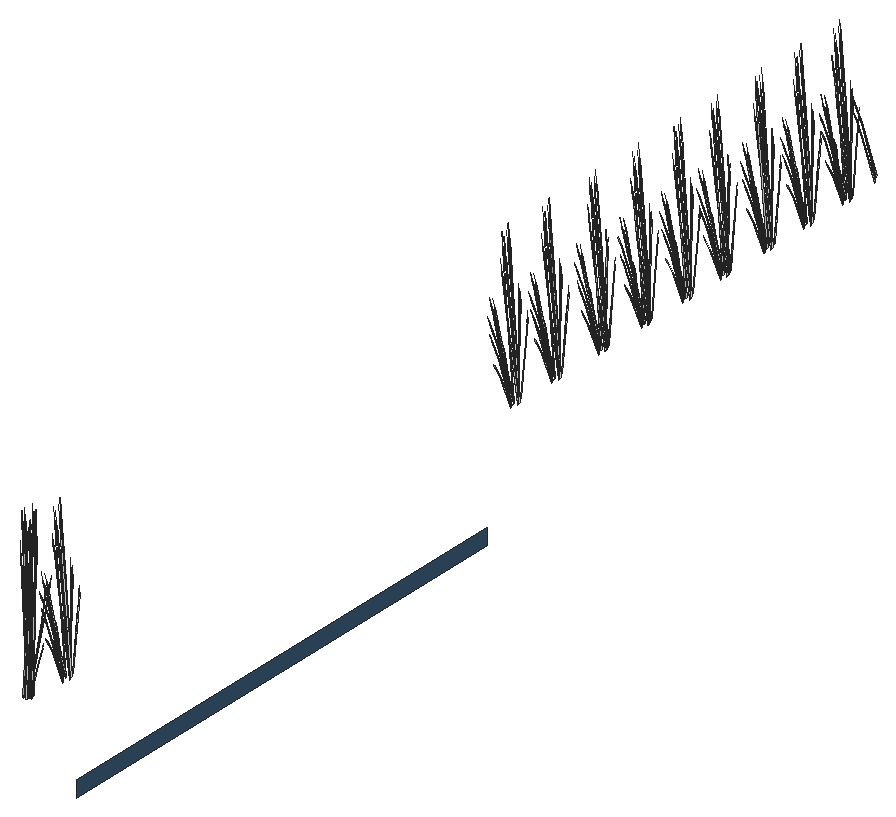
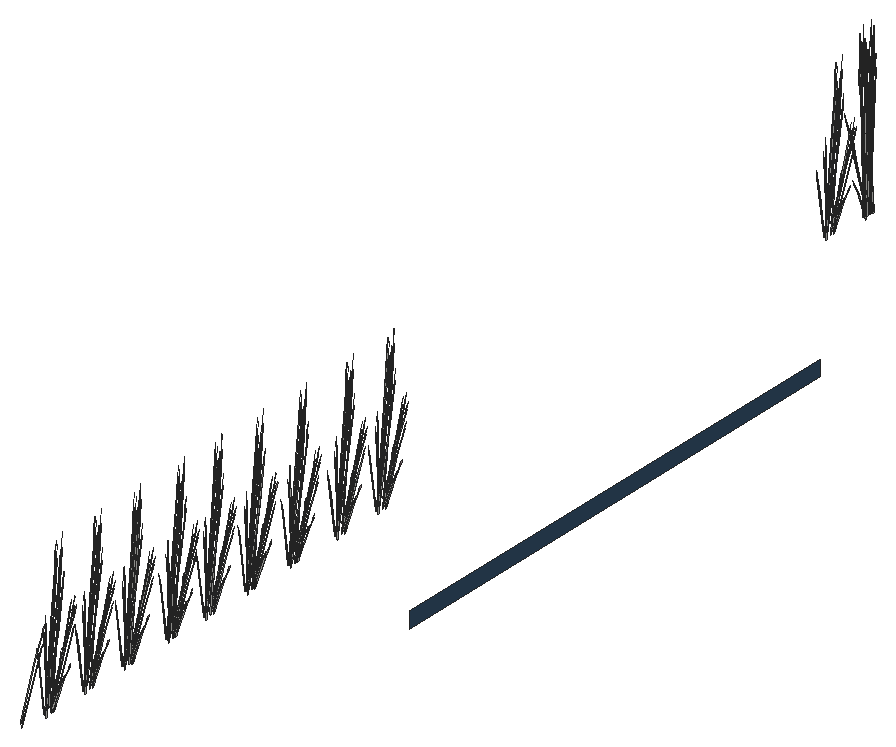
# SketchUp Ruby script. Lengths in inches.
U = 1.inch
M = Sketchup.active_model
def pt(a) = Geom::Point3d.new(a.map { |v| v * U })
def face(e, loops, mat)
  f = e.add_face(loops[0].map { |a| pt(a) })
  loops[1..].each { |l| e.add_face(l.map { |a| pt(a) }).erase! }
  f.material = f.back_material = mat if mat
  f
end
# faces: each face lists its corners as indices into pts; further lists are holes
def faces(e, pts, list, mat = nil) = list.each { |f| face(e, (f[0].is_a?(Array) ? f : [f]).map { |l| l.map { |i| pts[i] } }, mat) }
# xy, xz, yz: faces in a plane at the given z, y or x. An outline is a flat list of corners, or four numbers for a rectangle; further outlines are holes
def ring(l) = l.size == 4 ? [[l[0], l[1]], [l[2], l[1]], [l[2], l[3]], [l[0], l[3]]] : l.each_slice(2).to_a
def flat(e, list, mat, &to3) = list.each { |f| face(e, (f[0].is_a?(Array) ? f : [f]).map { |l| ring(l).map { |u, v| to3.(u, v) } }, mat) }
def xy(e, z, list, mat = nil) = flat(e, list, mat) { |x, y| [x, y, z] }
def xz(e, y, list, mat = nil) = flat(e, list, mat) { |x, z| [x, y, z] }
def yz(e, x, list, mat = nil) = flat(e, list, mat) { |y, z| [x, y, z] }
def lines(e, pts, list) = list.each { |a, b| e.add_line(pt(pts[a]), pt(pts[b])) }
# prism: a flat outline (further loops are holes) pulled along v
def prism(e, loops, v, mat = nil)
  f = face(e, loops, mat); d = Geom::Vector3d.new(v.map { |x| x * U })
  f.pushpull(f.normal.samedirection?(d) ? d.length : -d.length)
end
def box(e, o, s, mat = nil) = prism(e, [[o, [o[0] + s[0], o[1], o[2]], [o[0] + s[0], o[1] + s[1], o[2]], [o[0], o[1] + s[1], o[2]]]], [0, 0, s[2]], mat)
def at(x, y, z, deg = 0) = Geom::Transformation.translation(pt([x, y, z])) * Geom::Transformation.rotation(ORIGIN, Z_AXIS, deg.degrees)
def axes(o, x, y, z) = Geom::Transformation.new([*x, 0, *y, 0, *z, 0, *pt(o).to_a, 1])
def part(name) = M.definitions.add(name)
# library, detail: a bought-in or finely detailed component or shape, given as its bounding box
def library(name, o, s) = part(name).tap { |d| box(d.entities, o, s) }
def detail(e, o, s) = box(e.add_group.entities, o, s)
def put(e, d, t, mat = nil) = e.add_instance(d, t).tap { |i| i.material = mat if mat }
def group(e, t, mat = nil) = e.add_group.tap { |g| g.transformation = t; g.material = mat if mat }.entities
root = M.entities
M.materials.add("Carpet_04_1K").color = [56, 85, 112]
M.materials.add("LightPink_Translucent").color = [144, 107, 117]
M.materials["LightPink_Translucent"].alpha = 0.75
c1 = part("blade")
p = [[2.15,0.21,22],[0,0.17,0],[0.09,0.45,0],[2.18,0.31,22],[2.29,0.31,22],[0.38,0.45,0],
  [2.48,0.24,33],[2.49,0.24,33],[2.48,0.22,33]]
faces(c1.entities,p,[[0,1,2,3],[4,5,2,3],[6,3,4,7],[8,0,3,6]])
c2 = part("seeds")
p = [[0.3,-0.1,1.38],[-0.01,-0.03,1.59],[-0.01,-0.03,0.03],[0.14,-0.07,-0.07],[0.29,-0.03,3],[0.15,0.01,3.11]]
faces(c2.entities,p,[[0,1,2,3],[1,0,4,5]],"LightPink_Translucent")
c3 = part("blade with seeds")
put(c3.entities,c1,at(0,0,0))
put(c3.entities,c2,axes([2.4,0.25,30.99],[1.5799,-0.05474,1.17369],[-0.12525,1.92788,0.29478],[-0.07173,-0.02425,1.56792]))
yz(root,398.57,[[316.3,-42,509.26,-36]],"Carpet_04_1K")
put(root,c3,axes([400.43,618.83,4.53],[-0.30722,0.06665,-0.35414],[-0.08112,-0.381,0.4572],[-0.08804,0.10234,0.87481]))
put(root,c3,axes([400.43,639.36,4.53],[-0.30722,0.06665,-0.35414],[-0.08112,-0.381,0.4572],[-0.08804,0.10234,0.87481]))
put(root,c3,axes([400.43,658.04,4.53],[-0.30722,0.06665,-0.35414],[-0.08112,-0.381,0.4572],[-0.08804,0.10234,0.87481]))
put(root,c3,axes([400.43,676.25,4.53],[-0.30722,0.06665,-0.35414],[-0.08112,-0.381,0.4572],[-0.08804,0.10234,0.87481]))
put(root,c3,axes([398.73,292.91,2.72],[-0.17124,0.42022,0.44739],[-0.35581,-0.20224,-0.21531],[0,-0.09687,1.43643]))
put(root,c3,axes([400.27,311.16,1.49],[0.04734,0.04659,1.76342],[0.08027,0.4317,-0.26939],[-0.10492,0.09206,0.30037]))
put(root,c3,axes([400.27,521.6,1.49],[0.04734,0.04659,1.76342],[0.08027,0.4317,-0.26939],[-0.10492,0.09206,0.30037]))
put(root,c3,axes([400.27,540.83,1.49],[0.04734,0.04659,1.76342],[0.08027,0.4317,-0.26939],[-0.10492,0.09206,0.30037]))
put(root,c3,axes([400.27,562.67,1.49],[0.04734,0.04659,1.76342],[0.08027,0.4317,-0.26939],[-0.10492,0.09206,0.30037]))
put(root,c3,axes([400.27,582.9375,1.49],[0.04734,0.04659,1.76342],[0.08027,0.4317,-0.26939],[-0.10492,0.09206,0.30037]))
put(root,c3,axes([400.27,602.375,1.49],[0.04734,0.04659,1.76342],[0.08027,0.4317,-0.26939],[-0.10492,0.09206,0.30037]))
put(root,c3,axes([400.27,619.96,1.49],[0.04734,0.04659,1.76342],[0.08027,0.4317,-0.26939],[-0.10492,0.09206,0.30037]))
put(root,c3,axes([400.27,640.49,1.49],[0.04734,0.04659,1.76342],[0.08027,0.4317,-0.26939],[-0.10492,0.09206,0.30037]))
put(root,c3,axes([400.27,659.17,1.49],[0.04734,0.04659,1.76342],[0.08027,0.4317,-0.26939],[-0.10492,0.09206,0.30037]))
put(root,c3,axes([400.27,677.38,1.49],[0.04734,0.04659,1.76342],[0.08027,0.4317,-0.26939],[-0.10492,0.09206,0.30037]))
put(root,c3,axes([400.2,308.625,2.77],[0.22533,-0.03337,1.1486],[-0.14293,0.29403,0.84392],[-0.11135,-0.04411,0.25299]))
put(root,c3,axes([400.2,519.06,2.77],[0.22533,-0.03337,1.1486],[-0.14293,0.29403,0.84392],[-0.11135,-0.04411,0.25299]))
put(root,c3,axes([400.2,538.29,2.77],[0.22533,-0.03337,1.1486],[-0.14293,0.29403,0.84392],[-0.11135,-0.04411,0.25299]))
put(root,c3,axes([400.2,560.13,2.77],[0.22533,-0.03337,1.1486],[-0.14293,0.29403,0.84392],[-0.11135,-0.04411,0.25299]))
put(root,c3,axes([400.2,580.4,2.77],[0.22533,-0.03337,1.1486],[-0.14293,0.29403,0.84392],[-0.11135,-0.04411,0.25299]))
put(root,c3,axes([400.2,599.84,2.77],[0.22533,-0.03337,1.1486],[-0.14293,0.29403,0.84392],[-0.11135,-0.04411,0.25299]))
put(root,c3,axes([400.2,617.42,2.77],[0.22533,-0.03337,1.1486],[-0.14293,0.29403,0.84392],[-0.11135,-0.04411,0.25299]))
put(root,c3,axes([400.2,637.95,2.77],[0.22533,-0.03337,1.1486],[-0.14293,0.29403,0.84392],[-0.11135,-0.04411,0.25299]))
put(root,c3,axes([400.2,656.63,2.77],[0.22533,-0.03337,1.1486],[-0.14293,0.29403,0.84392],[-0.11135,-0.04411,0.25299]))
put(root,c3,axes([400.2,674.84,2.77],[0.22533,-0.03337,1.1486],[-0.14293,0.29403,0.84392],[-0.11135,-0.04411,0.25299]))
put(root,c3,axes([398.61,293.9,2.47],[0.37926,-0.12378,0.17642],[0.09365,0.46065,0.35086],[-0.03382,-0.06712,1.60407]))
put(root,c3,axes([399.1,293.98,2.2],[-0.35581,-0.20937,0],[0.17124,-0.43505,0],[0,0,1.62707]))
put(root,c3,axes([399.92,294.5,2.375],[0.22066,0.46731,0],[-0.36918,0.26061,-0.51607],[-0.08408,0.05936,1.63711]))
put(root,c3,axes([399.74,293.93,2.47],[0.10196,-0.46348,0.17642],[0.3731,0.13116,0.35086],[-0.06445,0.00226,1.60407]))
put(root,c3,axes([400.9,310.01,3.875],[0.06572,-0.16029,1.71376],[0.27569,0.33172,0.13857],[-0.12437,0.20675,0.73262]))
put(root,c3,axes([400.9,520.45,3.875],[0.06572,-0.16029,1.71376],[0.27569,0.33172,0.13857],[-0.12437,0.20675,0.73262]))
put(root,c3,axes([400.9,539.67,3.875],[0.06572,-0.16029,1.71376],[0.27569,0.33172,0.13857],[-0.12437,0.20675,0.73262]))
put(root,c3,axes([400.9,561.52,3.875],[0.06572,-0.16029,1.71376],[0.27569,0.33172,0.13857],[-0.12437,0.20675,0.73262]))
put(root,c3,axes([400.9,581.79,3.875],[0.06572,-0.16029,1.71376],[0.27569,0.33172,0.13857],[-0.12437,0.20675,0.73262]))
put(root,c3,axes([400.9,601.22,3.875],[0.06572,-0.16029,1.71376],[0.27569,0.33172,0.13857],[-0.12437,0.20675,0.73262]))
put(root,c3,axes([400.9,618.81,3.875],[0.06572,-0.16029,1.71376],[0.27569,0.33172,0.13857],[-0.12437,0.20675,0.73262]))
put(root,c3,axes([400.9,639.34,3.875],[0.06572,-0.16029,1.71376],[0.27569,0.33172,0.13857],[-0.12437,0.20675,0.73262]))
put(root,c3,axes([400.9,658.02,3.875],[0.06572,-0.16029,1.71376],[0.27569,0.33172,0.13857],[-0.12437,0.20675,0.73262]))
put(root,c3,axes([400.9,676.23,3.875],[0.06572,-0.16029,1.71376],[0.27569,0.33172,0.13857],[-0.12437,0.20675,0.73262]))
put(root,c3,axes([399.57,293.3125,2.62],[0.26075,0.2802,0.1448],[-0.2175,0.31612,-0.41347],[-0.06054,0.04274,1.26744]))
put(root,c3,axes([399.47,292.97,2.3],[-0.32829,-0.4014,-0.06131],[0.32849,-0.40164,0],[-0.01146,-0.01402,1.75571]))
put(root,c3,axes([399.56,293.11,2.72],[0.38326,-0.02879,0.44739],[0.03466,0.47788,-0.21531],[-0.06861,0.04843,1.43643]))
put(root,c3,axes([399.65,294.21,2.33],[0.44186,0.15158,0.30756],[-0.11054,0.54181,-0.36492],[-0.07313,0.06781,1.64885]))
put(root,c3,axes([400.6875,310.08,4.68],[0.09067,0.42583,-0.51099],[-0.34336,0.07449,-0.3958],[-0.0984,0.11438,0.97773]))
put(root,c3,axes([400.6875,520.51,4.68],[0.09067,0.42583,-0.51099],[-0.34336,0.07449,-0.3958],[-0.0984,0.11438,0.97773]))
put(root,c3,axes([400.6875,539.74,4.68],[0.09067,0.42583,-0.51099],[-0.34336,0.07449,-0.3958],[-0.0984,0.11438,0.97773]))
put(root,c3,axes([400.6875,561.59,4.68],[0.09067,0.42583,-0.51099],[-0.34336,0.07449,-0.3958],[-0.0984,0.11438,0.97773]))
put(root,c3,axes([400.6875,581.85,4.68],[0.09067,0.42583,-0.51099],[-0.34336,0.07449,-0.3958],[-0.0984,0.11438,0.97773]))
put(root,c3,axes([400.6875,601.29,4.68],[0.09067,0.42583,-0.51099],[-0.34336,0.07449,-0.3958],[-0.0984,0.11438,0.97773]))
put(root,c3,axes([400.6875,618.87,4.68],[0.09067,0.42583,-0.51099],[-0.34336,0.07449,-0.3958],[-0.0984,0.11438,0.97773]))
put(root,c3,axes([400.6875,639.41,4.68],[0.09067,0.42583,-0.51099],[-0.34336,0.07449,-0.3958],[-0.0984,0.11438,0.97773]))
put(root,c3,axes([400.6875,658.08,4.68],[0.09067,0.42583,-0.51099],[-0.34336,0.07449,-0.3958],[-0.0984,0.11438,0.97773]))
put(root,c3,axes([400.6875,676.3,4.68],[0.09067,0.42583,-0.51099],[-0.34336,0.07449,-0.3958],[-0.0984,0.11438,0.97773]))
put(root,c3,axes([399.84,294.18,2.48],[0.33032,-0.23318,0.49651],[0.19744,0.41812,0],[-0.07523,0.05311,1.57504]))
put(root,c3,axes([398.81,292.5,2.36],[0.15345,0.52148,0.45755],[-0.43845,0.18134,0.17955],[0.00536,-0.09582,1.58856]))
put(root,c3,axes([401.54,309.77,2.06],[-0.36714,-0.07646,-0.62353],[0.07747,-0.47163,-0.16365],[-0.10956,-0.05715,1.37633]))
put(root,c3,axes([401.54,520.21,2.06],[-0.36714,-0.07646,-0.62353],[0.07747,-0.47163,-0.16365],[-0.10956,-0.05715,1.37633]))
put(root,c3,axes([401.54,539.43,2.06],[-0.36714,-0.07646,-0.62353],[0.07747,-0.47163,-0.16365],[-0.10956,-0.05715,1.37633]))
put(root,c3,axes([401.54,561.28,2.06],[-0.36714,-0.07646,-0.62353],[0.07747,-0.47163,-0.16365],[-0.10956,-0.05715,1.37633]))
put(root,c3,axes([401.54,581.55,2.06],[-0.36714,-0.07646,-0.62353],[0.07747,-0.47163,-0.16365],[-0.10956,-0.05715,1.37633]))
put(root,c3,axes([401.54,600.98,2.06],[-0.36714,-0.07646,-0.62353],[0.07747,-0.47163,-0.16365],[-0.10956,-0.05715,1.37633]))
put(root,c3,axes([401.54,618.57,2.06],[-0.36714,-0.07646,-0.62353],[0.07747,-0.47163,-0.16365],[-0.10956,-0.05715,1.37633]))
put(root,c3,axes([401.54,639.1,2.06],[-0.36714,-0.07646,-0.62353],[0.07747,-0.47163,-0.16365],[-0.10956,-0.05715,1.37633]))
put(root,c3,axes([401.54,657.78,2.06],[-0.36714,-0.07646,-0.62353],[0.07747,-0.47163,-0.16365],[-0.10956,-0.05715,1.37633]))
put(root,c3,axes([401.54,675.99,2.06],[-0.36714,-0.07646,-0.62353],[0.07747,-0.47163,-0.16365],[-0.10956,-0.05715,1.37633]))
put(root,c3,axes([399.18,293.79,2.2],[-0.11516,-0.40207,0],[0.32884,-0.1408,0],[0,0,1.54371]))
put(root,c3,axes([398.76,294.64,1.49],[0.05712,-0.02538,1.76342],[0.34359,0.13968,-0.26939],[0.01005,0.15742,0.30037]))
put(root,c3,axes([398.84,294.78,4.53],[-0.1064,0.35863,-0.35414],[-0.31043,-0.1046,0.4572],[0.02846,0.14439,0.87481]))
put(root,c3,axes([401.51,307.5625,4.98],[-0.30095,-0.22541,-0.71045],[0.21388,-0.395,0.08574],[-0.10904,-0.13459,1.00501]))
put(root,c3,axes([401.51,518,4.98],[-0.30095,-0.22541,-0.71045],[0.21388,-0.395,0.08574],[-0.10904,-0.13459,1.00501]))
put(root,c3,axes([401.51,537.23,4.98],[-0.30095,-0.22541,-0.71045],[0.21388,-0.395,0.08574],[-0.10904,-0.13459,1.00501]))
put(root,c3,axes([401.51,559.07,4.98],[-0.30095,-0.22541,-0.71045],[0.21388,-0.395,0.08574],[-0.10904,-0.13459,1.00501]))
put(root,c3,axes([401.51,579.34,4.98],[-0.30095,-0.22541,-0.71045],[0.21388,-0.395,0.08574],[-0.10904,-0.13459,1.00501]))
put(root,c3,axes([401.51,598.77,4.98],[-0.30095,-0.22541,-0.71045],[0.21388,-0.395,0.08574],[-0.10904,-0.13459,1.00501]))
put(root,c3,axes([401.51,616.36,4.98],[-0.30095,-0.22541,-0.71045],[0.21388,-0.395,0.08574],[-0.10904,-0.13459,1.00501]))
put(root,c3,axes([401.51,636.89,4.98],[-0.30095,-0.22541,-0.71045],[0.21388,-0.395,0.08574],[-0.10904,-0.13459,1.00501]))
put(root,c3,axes([401.51,655.57,4.98],[-0.30095,-0.22541,-0.71045],[0.21388,-0.395,0.08574],[-0.10904,-0.13459,1.00501]))
put(root,c3,axes([401.51,673.78,4.98],[-0.30095,-0.22541,-0.71045],[0.21388,-0.395,0.08574],[-0.10904,-0.13459,1.00501]))
put(root,c3,axes([401.37,307.57,4.68],[-0.34827,0.11086,-0.51099],[-0.06092,-0.41983,-0.3958],[-0.09354,-0.12031,0.97773]))
put(root,c3,axes([401.37,518.01,4.68],[-0.34827,0.11086,-0.51099],[-0.06092,-0.41983,-0.3958],[-0.09354,-0.12031,0.97773]))
put(root,c3,axes([401.37,537.24,4.68],[-0.34827,0.11086,-0.51099],[-0.06092,-0.41983,-0.3958],[-0.09354,-0.12031,0.97773]))
put(root,c3,axes([401.37,559.08,4.68],[-0.34827,0.11086,-0.51099],[-0.06092,-0.41983,-0.3958],[-0.09354,-0.12031,0.97773]))
put(root,c3,axes([401.37,579.35,4.68],[-0.34827,0.11086,-0.51099],[-0.06092,-0.41983,-0.3958],[-0.09354,-0.12031,0.97773]))
put(root,c3,axes([401.37,598.79,4.68],[-0.34827,0.11086,-0.51099],[-0.06092,-0.41983,-0.3958],[-0.09354,-0.12031,0.97773]))
put(root,c3,axes([401.37,616.37,4.68],[-0.34827,0.11086,-0.51099],[-0.06092,-0.41983,-0.3958],[-0.09354,-0.12031,0.97773]))
put(root,c3,axes([401.37,636.9,4.68],[-0.34827,0.11086,-0.51099],[-0.06092,-0.41983,-0.3958],[-0.09354,-0.12031,0.97773]))
put(root,c3,axes([401.37,655.58,4.68],[-0.34827,0.11086,-0.51099],[-0.06092,-0.41983,-0.3958],[-0.09354,-0.12031,0.97773]))
put(root,c3,axes([401.37,673.79,4.68],[-0.34827,0.11086,-0.51099],[-0.06092,-0.41983,-0.3958],[-0.09354,-0.12031,0.97773]))
put(root,c3,axes([401.0625,310.66,2.02],[-0.33032,-0.23318,-0.49651],[0.19744,-0.41812,0],[-0.07523,-0.05311,1.57504]))
put(root,c3,axes([401.0625,521.1,2.02],[-0.33032,-0.23318,-0.49651],[0.19744,-0.41812,0],[-0.07523,-0.05311,1.57504]))
put(root,c3,axes([401.0625,540.33,2.02],[-0.33032,-0.23318,-0.49651],[0.19744,-0.41812,0],[-0.07523,-0.05311,1.57504]))
put(root,c3,axes([401.0625,562.17,2.02],[-0.33032,-0.23318,-0.49651],[0.19744,-0.41812,0],[-0.07523,-0.05311,1.57504]))
put(root,c3,axes([401.0625,582.44,2.02],[-0.33032,-0.23318,-0.49651],[0.19744,-0.41812,0],[-0.07523,-0.05311,1.57504]))
put(root,c3,axes([401.0625,601.875,2.02],[-0.33032,-0.23318,-0.49651],[0.19744,-0.41812,0],[-0.07523,-0.05311,1.57504]))
put(root,c3,axes([401.0625,619.46,2.02],[-0.33032,-0.23318,-0.49651],[0.19744,-0.41812,0],[-0.07523,-0.05311,1.57504]))
put(root,c3,axes([401.0625,639.99,2.02],[-0.33032,-0.23318,-0.49651],[0.19744,-0.41812,0],[-0.07523,-0.05311,1.57504]))
put(root,c3,axes([401.0625,658.67,2.02],[-0.33032,-0.23318,-0.49651],[0.19744,-0.41812,0],[-0.07523,-0.05311,1.57504]))
put(root,c3,axes([401.0625,676.88,2.02],[-0.33032,-0.23318,-0.49651],[0.19744,-0.41812,0],[-0.07523,-0.05311,1.57504]))
put(root,c3,axes([400.92,307.19,1.49],[-0.03419,0.06144,1.76342],[-0.3455,0.13246,-0.26939],[-0.08346,-0.12049,0.30037]))
put(root,c3,axes([400.92,517.625,1.49],[-0.03419,0.06144,1.76342],[-0.3455,0.13246,-0.26939],[-0.08346,-0.12049,0.30037]))
put(root,c3,axes([400.92,536.85,1.49],[-0.03419,0.06144,1.76342],[-0.3455,0.13246,-0.26939],[-0.08346,-0.12049,0.30037]))
put(root,c3,axes([400.92,558.7,1.49],[-0.03419,0.06144,1.76342],[-0.3455,0.13246,-0.26939],[-0.08346,-0.12049,0.30037]))
put(root,c3,axes([400.92,578.97,1.49],[-0.03419,0.06144,1.76342],[-0.3455,0.13246,-0.26939],[-0.08346,-0.12049,0.30037]))
put(root,c3,axes([400.92,598.4,1.49],[-0.03419,0.06144,1.76342],[-0.3455,0.13246,-0.26939],[-0.08346,-0.12049,0.30037]))
put(root,c3,axes([400.92,615.99,1.49],[-0.03419,0.06144,1.76342],[-0.3455,0.13246,-0.26939],[-0.08346,-0.12049,0.30037]))
put(root,c3,axes([400.92,636.52,1.49],[-0.03419,0.06144,1.76342],[-0.3455,0.13246,-0.26939],[-0.08346,-0.12049,0.30037]))
put(root,c3,axes([400.92,655.2,1.49],[-0.03419,0.06144,1.76342],[-0.3455,0.13246,-0.26939],[-0.08346,-0.12049,0.30037]))
put(root,c3,axes([400.92,673.41,1.49],[-0.03419,0.06144,1.76342],[-0.3455,0.13246,-0.26939],[-0.08346,-0.12049,0.30037]))
put(root,c3,axes([399.64,293,2.21],[-0.17124,0.42022,-0.44739],[-0.35581,-0.20224,0.21531],[0,0.09687,1.43643]))
put(root,c3,axes([401.26,310.95,2.375],[-0.22066,0.46731,0],[-0.36918,-0.26061,-0.51607],[-0.08408,-0.05936,1.63711]))
put(root,c3,axes([401.26,521.38,2.375],[-0.22066,0.46731,0],[-0.36918,-0.26061,-0.51607],[-0.08408,-0.05936,1.63711]))
put(root,c3,axes([401.26,540.61,2.375],[-0.22066,0.46731,0],[-0.36918,-0.26061,-0.51607],[-0.08408,-0.05936,1.63711]))
put(root,c3,axes([401.26,562.45,2.375],[-0.22066,0.46731,0],[-0.36918,-0.26061,-0.51607],[-0.08408,-0.05936,1.63711]))
put(root,c3,axes([401.26,582.72,2.375],[-0.22066,0.46731,0],[-0.36918,-0.26061,-0.51607],[-0.08408,-0.05936,1.63711]))
put(root,c3,axes([401.26,602.16,2.375],[-0.22066,0.46731,0],[-0.36918,-0.26061,-0.51607],[-0.08408,-0.05936,1.63711]))
put(root,c3,axes([401.26,619.74,2.375],[-0.22066,0.46731,0],[-0.36918,-0.26061,-0.51607],[-0.08408,-0.05936,1.63711]))
put(root,c3,axes([401.26,640.28,2.375],[-0.22066,0.46731,0],[-0.36918,-0.26061,-0.51607],[-0.08408,-0.05936,1.63711]))
put(root,c3,axes([401.26,658.95,2.375],[-0.22066,0.46731,0],[-0.36918,-0.26061,-0.51607],[-0.08408,-0.05936,1.63711]))
put(root,c3,axes([401.26,677.17,2.375],[-0.22066,0.46731,0],[-0.36918,-0.26061,-0.51607],[-0.08408,-0.05936,1.63711]))
put(root,c3,axes([400.32,292.74,2.47],[-0.2773,-0.3397,0.17642],[0.27945,-0.32949,0.35086],[-0.03063,0.06937,1.60407]))
put(root,c3,axes([399.36,292.55,2.21],[0,-0.53961,0],[0.44133,0,0],[0,0,1.79456]))
put(root,c3,axes([399.58,292.76,2.29],[0,0.53934,-0.05637],[-0.44133,0,0],[0,0.01695,1.79368]))
put(root,c3,axes([398.64,291.51,2.47],[-0.10196,0.46348,0.17642],[-0.3731,-0.13116,0.35086],[0.06445,-0.00226,1.60407]))
put(root,c3,axes([400.86,311.62,2.59],[0.11138,-0.07357,1.43002],[0.27499,0.22183,-0.30754],[-0.08185,0.19194,0.61141]))
put(root,c3,axes([400.86,522.06,2.59],[0.11138,-0.07357,1.43002],[0.27499,0.22183,-0.30754],[-0.08185,0.19194,0.61141]))
put(root,c3,axes([400.86,541.29,2.59],[0.11138,-0.07357,1.43002],[0.27499,0.22183,-0.30754],[-0.08185,0.19194,0.61141]))
put(root,c3,axes([400.86,563.13,2.59],[0.11138,-0.07357,1.43002],[0.27499,0.22183,-0.30754],[-0.08185,0.19194,0.61141]))
put(root,c3,axes([400.86,583.4,2.59],[0.11138,-0.07357,1.43002],[0.27499,0.22183,-0.30754],[-0.08185,0.19194,0.61141]))
put(root,c3,axes([400.86,602.83,2.59],[0.11138,-0.07357,1.43002],[0.27499,0.22183,-0.30754],[-0.08185,0.19194,0.61141]))
put(root,c3,axes([400.86,620.42,2.59],[0.11138,-0.07357,1.43002],[0.27499,0.22183,-0.30754],[-0.08185,0.19194,0.61141]))
put(root,c3,axes([400.86,640.95,2.59],[0.11138,-0.07357,1.43002],[0.27499,0.22183,-0.30754],[-0.08185,0.19194,0.61141]))
put(root,c3,axes([400.86,659.625,2.59],[0.11138,-0.07357,1.43002],[0.27499,0.22183,-0.30754],[-0.08185,0.19194,0.61141]))
put(root,c3,axes([400.86,677.84,2.59],[0.11138,-0.07357,1.43002],[0.27499,0.22183,-0.30754],[-0.08185,0.19194,0.61141]))
put(root,c3,axes([399.37,293.81,2.29],[0.15345,0.53576,-0.06012],[-0.43845,0.18773,0],[0.00536,0.01871,1.72173]))
put(root,c3,axes([400.7,307.43,2.13],[-0.10181,0.3808,-0.03893],[-0.31336,-0.11714,-0.17649],[-0.04758,-0.06228,0.58215]))
put(root,c3,axes([400.7,517.86,2.13],[-0.10181,0.3808,-0.03893],[-0.31336,-0.11714,-0.17649],[-0.04758,-0.06228,0.58215]))
put(root,c3,axes([400.7,537.09,2.13],[-0.10181,0.3808,-0.03893],[-0.31336,-0.11714,-0.17649],[-0.04758,-0.06228,0.58215]))
put(root,c3,axes([400.7,558.9375,2.13],[-0.10181,0.3808,-0.03893],[-0.31336,-0.11714,-0.17649],[-0.04758,-0.06228,0.58215]))
put(root,c3,axes([400.7,579.2,2.13],[-0.10181,0.3808,-0.03893],[-0.31336,-0.11714,-0.17649],[-0.04758,-0.06228,0.58215]))
put(root,c3,axes([400.7,598.64,2.13],[-0.10181,0.3808,-0.03893],[-0.31336,-0.11714,-0.17649],[-0.04758,-0.06228,0.58215]))
put(root,c3,axes([400.7,616.22,2.13],[-0.10181,0.3808,-0.03893],[-0.31336,-0.11714,-0.17649],[-0.04758,-0.06228,0.58215]))
put(root,c3,axes([400.7,636.76,2.13],[-0.10181,0.3808,-0.03893],[-0.31336,-0.11714,-0.17649],[-0.04758,-0.06228,0.58215]))
put(root,c3,axes([400.7,655.43,2.13],[-0.10181,0.3808,-0.03893],[-0.31336,-0.11714,-0.17649],[-0.04758,-0.06228,0.58215]))
put(root,c3,axes([400.7,673.65,2.13],[-0.10181,0.3808,-0.03893],[-0.31336,-0.11714,-0.17649],[-0.04758,-0.06228,0.58215]))
put(root,c3,axes([398.87,294.46,4.98],[0.16845,0.3792,-0.71045],[-0.34676,0.21133,0.08574],[0.03939,0.18322,1.00501]))
put(root,c3,axes([400.64,293.1,2.2],[-0.44111,-0.00373,-0.04976],[0,-0.52122,0.49943],[-0.01386,0.11865,1.58352]))
put(root,c3,axes([401.17,306.95,2.59],[-0.02137,0.15256,1.43002],[-0.31245,0.12771,-0.30754],[-0.07303,-0.19719,0.61141]))
put(root,c3,axes([401.17,517.38,2.59],[-0.02137,0.15256,1.43002],[-0.31245,0.12771,-0.30754],[-0.07303,-0.19719,0.61141]))
put(root,c3,axes([401.17,536.61,2.59],[-0.02137,0.15256,1.43002],[-0.31245,0.12771,-0.30754],[-0.07303,-0.19719,0.61141]))
put(root,c3,axes([401.17,558.46,2.59],[-0.02137,0.15256,1.43002],[-0.31245,0.12771,-0.30754],[-0.07303,-0.19719,0.61141]))
put(root,c3,axes([401.17,578.72,2.59],[-0.02137,0.15256,1.43002],[-0.31245,0.12771,-0.30754],[-0.07303,-0.19719,0.61141]))
put(root,c3,axes([401.17,598.16,2.59],[-0.02137,0.15256,1.43002],[-0.31245,0.12771,-0.30754],[-0.07303,-0.19719,0.61141]))
put(root,c3,axes([401.17,615.74,2.59],[-0.02137,0.15256,1.43002],[-0.31245,0.12771,-0.30754],[-0.07303,-0.19719,0.61141]))
put(root,c3,axes([401.17,636.28,2.59],[-0.02137,0.15256,1.43002],[-0.31245,0.12771,-0.30754],[-0.07303,-0.19719,0.61141]))
put(root,c3,axes([401.17,654.95,2.59],[-0.02137,0.15256,1.43002],[-0.31245,0.12771,-0.30754],[-0.07303,-0.19719,0.61141]))
put(root,c3,axes([401.17,673.17,2.59],[-0.02137,0.15256,1.43002],[-0.31245,0.12771,-0.30754],[-0.07303,-0.19719,0.61141]))
put(root,c3,axes([401.17,688.24,2.59],[-0.02137,0.15256,1.43002],[-0.31245,0.12771,-0.30754],[-0.07303,-0.19719,0.61141]))
put(root,c3,axes([401.27,307.34,3.875],[0.08068,0.14973,1.71376],[-0.3728,0.12606,0.13857],[-0.08426,-0.23506,0.73262]))
put(root,c3,axes([401.27,517.78,3.875],[0.08068,0.14973,1.71376],[-0.3728,0.12606,0.13857],[-0.08426,-0.23506,0.73262]))
put(root,c3,axes([401.27,537.01,3.875],[0.08068,0.14973,1.71376],[-0.3728,0.12606,0.13857],[-0.08426,-0.23506,0.73262]))
put(root,c3,axes([401.27,558.85,3.875],[0.08068,0.14973,1.71376],[-0.3728,0.12606,0.13857],[-0.08426,-0.23506,0.73262]))
put(root,c3,axes([401.27,579.12,3.875],[0.08068,0.14973,1.71376],[-0.3728,0.12606,0.13857],[-0.08426,-0.23506,0.73262]))
put(root,c3,axes([401.27,598.56,3.875],[0.08068,0.14973,1.71376],[-0.3728,0.12606,0.13857],[-0.08426,-0.23506,0.73262]))
put(root,c3,axes([401.27,616.14,3.875],[0.08068,0.14973,1.71376],[-0.3728,0.12606,0.13857],[-0.08426,-0.23506,0.73262]))
put(root,c3,axes([401.27,636.67,3.875],[0.08068,0.14973,1.71376],[-0.3728,0.12606,0.13857],[-0.08426,-0.23506,0.73262]))
put(root,c3,axes([401.27,655.35,3.875],[0.08068,0.14973,1.71376],[-0.3728,0.12606,0.13857],[-0.08426,-0.23506,0.73262]))
put(root,c3,axes([401.27,673.5625,3.875],[0.08068,0.14973,1.71376],[-0.3728,0.12606,0.13857],[-0.08426,-0.23506,0.73262]))
put(root,c3,axes([401.27,688.64,3.875],[0.08068,0.14973,1.71376],[-0.3728,0.12606,0.13857],[-0.08426,-0.23506,0.73262]))
put(root,c3,axes([401.96,309.84,2.67],[-0.35635,0.30962,-0.29095],[-0.23697,-0.43749,-0.50002],[-0.08792,-0.04443,1.59708]))
put(root,c3,axes([401.96,520.28,2.67],[-0.35635,0.30962,-0.29095],[-0.23697,-0.43749,-0.50002],[-0.08792,-0.04443,1.59708]))
put(root,c3,axes([401.96,539.5,2.67],[-0.35635,0.30962,-0.29095],[-0.23697,-0.43749,-0.50002],[-0.08792,-0.04443,1.59708]))
put(root,c3,axes([401.96,561.35,2.67],[-0.35635,0.30962,-0.29095],[-0.23697,-0.43749,-0.50002],[-0.08792,-0.04443,1.59708]))
put(root,c3,axes([401.96,581.62,2.67],[-0.35635,0.30962,-0.29095],[-0.23697,-0.43749,-0.50002],[-0.08792,-0.04443,1.59708]))
put(root,c3,axes([401.96,601.05,2.67],[-0.35635,0.30962,-0.29095],[-0.23697,-0.43749,-0.50002],[-0.08792,-0.04443,1.59708]))
put(root,c3,axes([401.96,618.64,2.67],[-0.35635,0.30962,-0.29095],[-0.23697,-0.43749,-0.50002],[-0.08792,-0.04443,1.59708]))
put(root,c3,axes([401.96,639.17,2.67],[-0.35635,0.30962,-0.29095],[-0.23697,-0.43749,-0.50002],[-0.08792,-0.04443,1.59708]))
put(root,c3,axes([401.96,657.85,2.67],[-0.35635,0.30962,-0.29095],[-0.23697,-0.43749,-0.50002],[-0.08792,-0.04443,1.59708]))
put(root,c3,axes([401.96,676.0625,2.67],[-0.35635,0.30962,-0.29095],[-0.23697,-0.43749,-0.50002],[-0.08792,-0.04443,1.59708]))
put(root,c3,axes([399.77,291.54,2.47],[-0.37926,0.12378,0.17642],[-0.09365,-0.46065,0.35086],[0.03382,0.06712,1.60407]))
put(root,c3,axes([401.4,307.26,4.53],[-0.05451,-0.37564,-0.35414],[0.31161,-0.09919,0.4572],[-0.0837,-0.10765,0.87481]))
put(root,c3,axes([401.4,517.7,4.53],[-0.05451,-0.37564,-0.35414],[0.31161,-0.09919,0.4572],[-0.0837,-0.10765,0.87481]))
put(root,c3,axes([401.4,536.93,4.53],[-0.05451,-0.37564,-0.35414],[0.31161,-0.09919,0.4572],[-0.0837,-0.10765,0.87481]))
put(root,c3,axes([401.4,558.77,4.53],[-0.05451,-0.37564,-0.35414],[0.31161,-0.09919,0.4572],[-0.0837,-0.10765,0.87481]))
put(root,c3,axes([401.4,579.04,4.53],[-0.05451,-0.37564,-0.35414],[0.31161,-0.09919,0.4572],[-0.0837,-0.10765,0.87481]))
put(root,c3,axes([401.4,598.48,4.53],[-0.05451,-0.37564,-0.35414],[0.31161,-0.09919,0.4572],[-0.0837,-0.10765,0.87481]))
put(root,c3,axes([401.4,616.06,4.53],[-0.05451,-0.37564,-0.35414],[0.31161,-0.09919,0.4572],[-0.0837,-0.10765,0.87481]))
put(root,c3,axes([401.4,636.59,4.53],[-0.05451,-0.37564,-0.35414],[0.31161,-0.09919,0.4572],[-0.0837,-0.10765,0.87481]))
put(root,c3,axes([401.4,655.27,4.53],[-0.05451,-0.37564,-0.35414],[0.31161,-0.09919,0.4572],[-0.0837,-0.10765,0.87481]))
put(root,c3,axes([401.4,673.48,4.53],[-0.05451,-0.37564,-0.35414],[0.31161,-0.09919,0.4572],[-0.0837,-0.10765,0.87481]))
put(root,c3,axes([400.53,309.17,2.375],[-0.44133,0,0],[0,-0.52122,-0.51607],[0,-0.11871,1.63711]))
put(root,c3,axes([400.53,519.6,2.375],[-0.44133,0,0],[0,-0.52122,-0.51607],[0,-0.11871,1.63711]))
put(root,c3,axes([400.53,538.83,2.375],[-0.44133,0,0],[0,-0.52122,-0.51607],[0,-0.11871,1.63711]))
put(root,c3,axes([400.53,560.67,2.375],[-0.44133,0,0],[0,-0.52122,-0.51607],[0,-0.11871,1.63711]))
put(root,c3,axes([400.53,580.94,2.375],[-0.44133,0,0],[0,-0.52122,-0.51607],[0,-0.11871,1.63711]))
put(root,c3,axes([400.53,600.38,2.375],[-0.44133,0,0],[0,-0.52122,-0.51607],[0,-0.11871,1.63711]))
put(root,c3,axes([400.53,617.96,2.375],[-0.44133,0,0],[0,-0.52122,-0.51607],[0,-0.11871,1.63711]))
put(root,c3,axes([400.53,638.5,2.375],[-0.44133,0,0],[0,-0.52122,-0.51607],[0,-0.11871,1.63711]))
put(root,c3,axes([400.53,657.17,2.375],[-0.44133,0,0],[0,-0.52122,-0.51607],[0,-0.11871,1.63711]))
put(root,c3,axes([400.53,675.39,2.375],[-0.44133,0,0],[0,-0.52122,-0.51607],[0,-0.11871,1.63711]))
put(root,c3,axes([401.15,310.49,2.03],[-0.08291,-0.40636,-0.30978],[0.32928,-0.11539,0.30978],[-0.06638,-0.04686,1.38974]))
put(root,c3,axes([401.15,520.93,2.03],[-0.08291,-0.40636,-0.30978],[0.32928,-0.11539,0.30978],[-0.06638,-0.04686,1.38974]))
put(root,c3,axes([401.15,540.15,2.03],[-0.08291,-0.40636,-0.30978],[0.32928,-0.11539,0.30978],[-0.06638,-0.04686,1.38974]))
put(root,c3,axes([401.15,562,2.03],[-0.08291,-0.40636,-0.30978],[0.32928,-0.11539,0.30978],[-0.06638,-0.04686,1.38974]))
put(root,c3,axes([401.15,582.27,2.03],[-0.08291,-0.40636,-0.30978],[0.32928,-0.11539,0.30978],[-0.06638,-0.04686,1.38974]))
put(root,c3,axes([401.15,601.7,2.03],[-0.08291,-0.40636,-0.30978],[0.32928,-0.11539,0.30978],[-0.06638,-0.04686,1.38974]))
put(root,c3,axes([401.15,619.29,2.03],[-0.08291,-0.40636,-0.30978],[0.32928,-0.11539,0.30978],[-0.06638,-0.04686,1.38974]))
put(root,c3,axes([401.15,639.82,2.03],[-0.08291,-0.40636,-0.30978],[0.32928,-0.11539,0.30978],[-0.06638,-0.04686,1.38974]))
put(root,c3,axes([401.15,658.49,2.03],[-0.08291,-0.40636,-0.30978],[0.32928,-0.11539,0.30978],[-0.06638,-0.04686,1.38974]))
